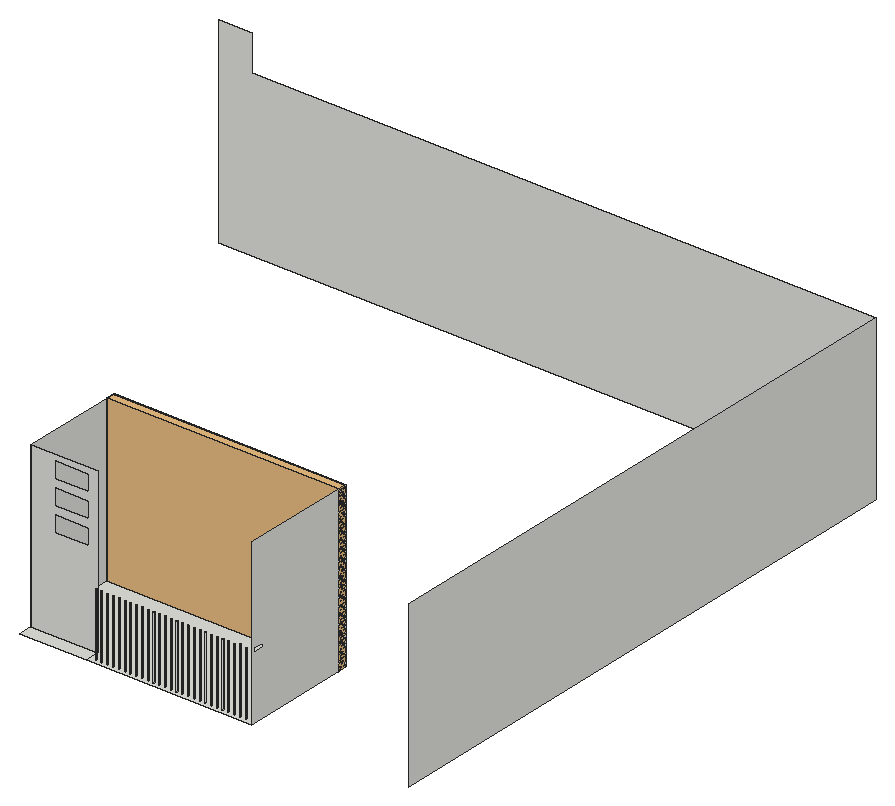
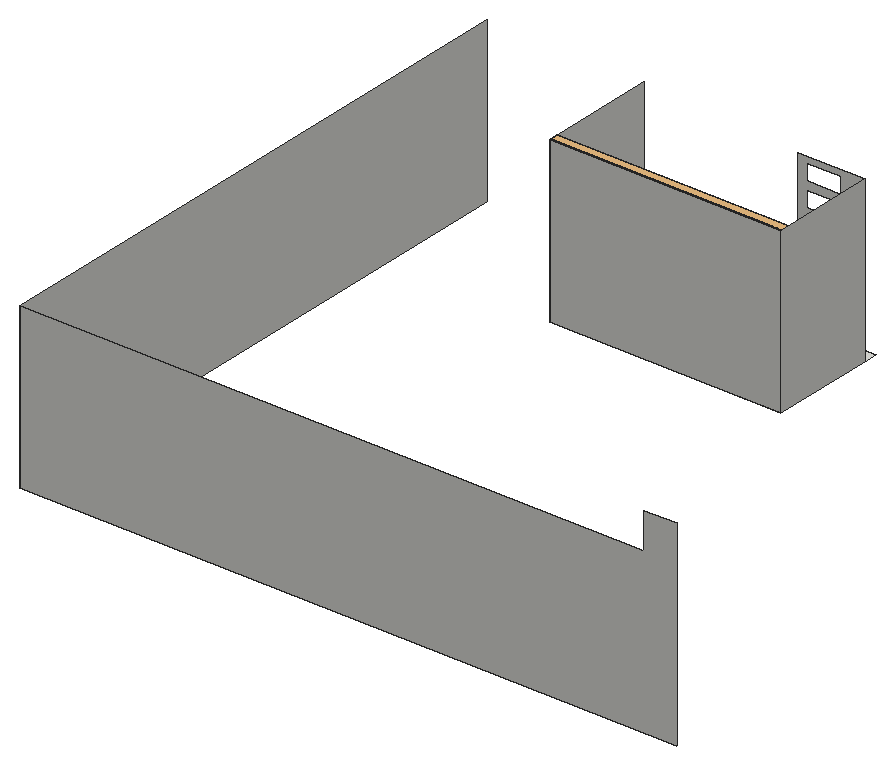
# SketchUp Ruby script. Lengths in inches.
U = 1.inch
M = Sketchup.active_model
def pt(a) = Geom::Point3d.new(a.map { |v| v * U })
def face(e, loops, mat)
  f = e.add_face(loops[0].map { |a| pt(a) })
  loops[1..].each { |l| e.add_face(l.map { |a| pt(a) }).erase! }
  f.material = f.back_material = mat if mat
  f
end
# faces: each face lists its corners as indices into pts; further lists are holes
def faces(e, pts, list, mat = nil) = list.each { |f| face(e, (f[0].is_a?(Array) ? f : [f]).map { |l| l.map { |i| pts[i] } }, mat) }
# xy, xz, yz: faces in a plane at the given z, y or x. An outline is a flat list of corners, or four numbers for a rectangle; further outlines are holes
def ring(l) = l.size == 4 ? [[l[0], l[1]], [l[2], l[1]], [l[2], l[3]], [l[0], l[3]]] : l.each_slice(2).to_a
def flat(e, list, mat, &to3) = list.each { |f| face(e, (f[0].is_a?(Array) ? f : [f]).map { |l| ring(l).map { |u, v| to3.(u, v) } }, mat) }
def xy(e, z, list, mat = nil) = flat(e, list, mat) { |x, y| [x, y, z] }
def xz(e, y, list, mat = nil) = flat(e, list, mat) { |x, z| [x, y, z] }
def yz(e, x, list, mat = nil) = flat(e, list, mat) { |y, z| [x, y, z] }
def lines(e, pts, list) = list.each { |a, b| e.add_line(pt(pts[a]), pt(pts[b])) }
# prism: a flat outline (further loops are holes) pulled along v
def prism(e, loops, v, mat = nil)
  f = face(e, loops, mat); d = Geom::Vector3d.new(v.map { |x| x * U })
  f.pushpull(f.normal.samedirection?(d) ? d.length : -d.length)
end
def box(e, o, s, mat = nil) = prism(e, [[o, [o[0] + s[0], o[1], o[2]], [o[0] + s[0], o[1] + s[1], o[2]], [o[0], o[1] + s[1], o[2]]]], [0, 0, s[2]], mat)
def at(x, y, z, deg = 0) = Geom::Transformation.translation(pt([x, y, z])) * Geom::Transformation.rotation(ORIGIN, Z_AXIS, deg.degrees)
def axes(o, x, y, z) = Geom::Transformation.new([*x, 0, *y, 0, *z, 0, *pt(o).to_a, 1])
def part(name) = M.definitions.add(name)
# library, detail: a bought-in or finely detailed component or shape, given as its bounding box
def library(name, o, s) = part(name).tap { |d| box(d.entities, o, s) }
def detail(e, o, s) = box(e.add_group.entities, o, s)
def put(e, d, t, mat = nil) = e.add_instance(d, t).tap { |i| i.material = mat if mat }
def group(e, t, mat = nil) = e.add_group.tap { |g| g.transformation = t; g.material = mat if mat }.entities
root = M.entities
c1 = library("Group\#10",[0,0,0],[238.3125,8.8125,168])
xy(root,819.75,[[290.4375,124.5,359.25,138.74],[[359.25,124.5,528.75,124.5,528.75,246,290.4375,246,290.4375,138.74,359.25,138.74],[370.76,127.81,370.55,127.83,370.35,127.91,370.1875,128.04,370.06,128.21,369.98,128.41,369.95,128.62,369.98,128.83,370.06,129.02,370.1875,129.19,370.35,129.32,370.55,129.4,370.76,129.43,370.97,129.4,371.17,129.32,371.34,129.19,371.46,129.02,371.55,128.83,371.57,128.62,371.55,128.41,371.46,128.21,371.34,128.04,371.17,127.91,370.97,127.83],[365.01,127.81,364.8,127.83,364.6,127.91,364.4375,128.04,364.31,128.21,364.23,128.41,364.2,128.62,364.23,128.83,364.31,129.02,364.4375,129.19,364.6,129.32,364.8,129.4,365.01,129.43,365.22,129.4,365.42,129.32,365.59,129.19,365.71,129.02,365.8,128.83,365.82,128.62,365.8,128.41,365.71,128.21,365.59,128.04,365.42,127.91,365.22,127.83],[376.7,127.81,376.49,127.83,376.29,127.91,376.125,128.04,375.99,128.21,375.91,128.41,375.89,128.62,375.91,128.83,375.99,129.02,376.125,129.19,376.29,129.32,376.49,129.4,376.7,129.43,376.91,129.4,377.1,129.32,377.27,129.19,377.4,129.02,377.48,128.83,377.51,128.62,377.48,128.41,377.4,128.21,377.27,128.04,377.1,127.91,376.91,127.83],[382.76,127.81,382.55,127.83,382.35,127.91,382.1875,128.04,382.06,128.21,381.98,128.41,381.95,128.62,381.98,128.83,382.06,129.02,382.1875,129.19,382.35,129.32,382.55,129.4,382.76,129.43,382.97,129.4,383.17,129.32,383.34,129.19,383.46,129.02,383.55,128.83,383.57,128.62,383.55,128.41,383.46,128.21,383.34,128.04,383.17,127.91,382.97,127.83],[388.82,127.81,388.61,127.83,388.42,127.91,388.25,128.04,388.12,128.21,388.04,128.41,388.01,128.62,388.04,128.83,388.12,129.02,388.25,129.19,388.42,129.32,388.61,129.4,388.82,129.43,389.03,129.4,389.23,129.32,389.4,129.19,389.53,129.02,389.61,128.83,389.64,128.62,389.61,128.41,389.53,128.21,389.4,128.04,389.23,127.91,389.03,127.83],[394.76,127.81,394.55,127.83,394.35,127.91,394.1875,128.04,394.06,128.21,393.98,128.41,393.95,128.62,393.98,128.83,394.06,129.02,394.1875,129.19,394.35,129.32,394.55,129.4,394.76,129.43,394.97,129.4,395.17,129.32,395.34,129.19,395.46,129.02,395.55,128.83,395.57,128.62,395.55,128.41,395.46,128.21,395.34,128.04,395.17,127.91,394.97,127.83],[400.57,127.81,400.36,127.83,400.17,127.91,400,128.04,399.87,128.21,399.79,128.41,399.76,128.62,399.79,128.83,399.87,129.02,400,129.19,400.17,129.32,400.36,129.4,400.57,129.43,400.78,129.4,400.98,129.32,401.15,129.19,401.28,129.02,401.36,128.83,401.39,128.62,401.36,128.41,401.28,128.21,401.15,128.04,400.98,127.91,400.78,127.83],[406.39,127.81,406.18,127.83,405.98,127.91,405.8125,128.04,405.68,128.21,405.6,128.41,405.57,128.62,405.6,128.83,405.68,129.02,405.8125,129.19,405.98,129.32,406.18,129.4,406.39,129.43,406.6,129.4,406.79,129.32,406.96,129.19,407.09,129.02,407.17,128.83,407.2,128.62,407.17,128.41,407.09,128.21,406.96,128.04,406.79,127.91,406.6,127.83],[412.32,127.81,412.11,127.83,411.92,127.91,411.75,128.04,411.62,128.21,411.54,128.41,411.51,128.62,411.54,128.83,411.62,129.02,411.75,129.19,411.92,129.32,412.11,129.4,412.32,129.43,412.53,129.4,412.73,129.32,412.9,129.19,413.03,129.02,413.11,128.83,413.14,128.62,413.11,128.41,413.03,128.21,412.9,128.04,412.73,127.91,412.53,127.83],[418.45,127.81,418.24,127.83,418.04,127.91,417.875,128.04,417.74,128.21,417.66,128.41,417.64,128.62,417.66,128.83,417.74,129.02,417.875,129.19,418.04,129.32,418.24,129.4,418.45,129.43,418.66,129.4,418.85,129.32,419.02,129.19,419.15,129.02,419.23,128.83,419.26,128.62,419.23,128.41,419.15,128.21,419.02,128.04,418.85,127.91,418.66,127.83],[424.39,127.81,424.18,127.83,423.98,127.91,423.8125,128.04,423.68,128.21,423.6,128.41,423.57,128.62,423.6,128.83,423.68,129.02,423.8125,129.19,423.98,129.32,424.18,129.4,424.39,129.43,424.6,129.4,424.79,129.32,424.96,129.19,425.09,129.02,425.17,128.83,425.2,128.62,425.17,128.41,425.09,128.21,424.96,128.04,424.79,127.91,424.6,127.83],[430.2,127.81,429.99,127.83,429.79,127.91,429.625,128.04,429.49,128.21,429.41,128.41,429.39,128.62,429.41,128.83,429.49,129.02,429.625,129.19,429.79,129.32,429.99,129.4,430.2,129.43,430.41,129.4,430.6,129.32,430.77,129.19,430.9,129.02,430.98,128.83,431.01,128.62,430.98,128.41,430.9,128.21,430.77,128.04,430.6,127.91,430.41,127.83],[436.01,127.81,435.8,127.83,435.6,127.91,435.4375,128.04,435.31,128.21,435.23,128.41,435.2,128.62,435.23,128.83,435.31,129.02,435.4375,129.19,435.6,129.32,435.8,129.4,436.01,129.43,436.22,129.4,436.42,129.32,436.59,129.19,436.71,129.02,436.8,128.83,436.82,128.62,436.8,128.41,436.71,128.21,436.59,128.04,436.42,127.91,436.22,127.83],[442.01,127.81,441.8,127.83,441.6,127.91,441.4375,128.04,441.31,128.21,441.23,128.41,441.2,128.62,441.23,128.83,441.31,129.02,441.4375,129.19,441.6,129.32,441.8,129.4,442.01,129.43,442.22,129.4,442.42,129.32,442.59,129.19,442.71,129.02,442.8,128.83,442.82,128.62,442.8,128.41,442.71,128.21,442.59,128.04,442.42,127.91,442.22,127.83],[448.07,127.81,447.86,127.83,447.67,127.91,447.5,128.04,447.37,128.21,447.29,128.41,447.26,128.62,447.29,128.83,447.37,129.02,447.5,129.19,447.67,129.32,447.86,129.4,448.07,129.43,448.28,129.4,448.48,129.32,448.65,129.19,448.78,129.02,448.86,128.83,448.89,128.62,448.86,128.41,448.78,128.21,448.65,128.04,448.48,127.91,448.28,127.83],[453.89,127.81,453.68,127.83,453.48,127.91,453.3125,128.04,453.18,128.21,453.1,128.41,453.07,128.62,453.1,128.83,453.18,129.02,453.3125,129.19,453.48,129.32,453.68,129.4,453.89,129.43,454.1,129.4,454.29,129.32,454.46,129.19,454.59,129.02,454.67,128.83,454.7,128.62,454.67,128.41,454.59,128.21,454.46,128.04,454.29,127.91,454.1,127.83],[459.95,127.81,459.74,127.83,459.54,127.91,459.375,128.04,459.24,128.21,459.16,128.41,459.14,128.62,459.16,128.83,459.24,129.02,459.375,129.19,459.54,129.32,459.74,129.4,459.95,129.43,460.16,129.4,460.35,129.32,460.52,129.19,460.65,129.02,460.73,128.83,460.76,128.62,460.73,128.41,460.65,128.21,460.52,128.04,460.35,127.91,460.16,127.83],[465.76,127.81,465.55,127.83,465.35,127.91,465.1875,128.04,465.06,128.21,464.98,128.41,464.95,128.62,464.98,128.83,465.06,129.02,465.1875,129.19,465.35,129.32,465.55,129.4,465.76,129.43,465.97,129.4,466.17,129.32,466.34,129.19,466.46,129.02,466.55,128.83,466.57,128.62,466.55,128.41,466.46,128.21,466.34,128.04,466.17,127.91,465.97,127.83],[471.95,127.81,471.74,127.83,471.54,127.91,471.375,128.04,471.24,128.21,471.16,128.41,471.14,128.62,471.16,128.83,471.24,129.02,471.375,129.19,471.54,129.32,471.74,129.4,471.95,129.43,472.16,129.4,472.35,129.32,472.52,129.19,472.65,129.02,472.73,128.83,472.76,128.62,472.73,128.41,472.65,128.21,472.52,128.04,472.35,127.91,472.16,127.83],[477.76,127.81,477.55,127.83,477.35,127.91,477.1875,128.04,477.06,128.21,476.98,128.41,476.95,128.62,476.98,128.83,477.06,129.02,477.1875,129.19,477.35,129.32,477.55,129.4,477.76,129.43,477.97,129.4,478.17,129.32,478.34,129.19,478.46,129.02,478.55,128.83,478.57,128.62,478.55,128.41,478.46,128.21,478.34,128.04,478.17,127.91,477.97,127.83],[483.76,127.81,483.55,127.83,483.35,127.91,483.1875,128.04,483.06,128.21,482.98,128.41,482.95,128.62,482.98,128.83,483.06,129.02,483.1875,129.19,483.35,129.32,483.55,129.4,483.76,129.43,483.97,129.4,484.17,129.32,484.34,129.19,484.46,129.02,484.55,128.83,484.57,128.62,484.55,128.41,484.46,128.21,484.34,128.04,484.17,127.91,483.97,127.83],[489.89,127.81,489.68,127.83,489.48,127.91,489.3125,128.04,489.18,128.21,489.1,128.41,489.07,128.62,489.1,128.83,489.18,129.02,489.3125,129.19,489.48,129.32,489.68,129.4,489.89,129.43,490.1,129.4,490.29,129.32,490.46,129.19,490.59,129.02,490.67,128.83,490.7,128.62,490.67,128.41,490.59,128.21,490.46,128.04,490.29,127.91,490.1,127.83],[495.39,127.81,495.18,127.83,494.98,127.91,494.8125,128.04,494.68,128.21,494.6,128.41,494.57,128.62,494.6,128.83,494.68,129.02,494.8125,129.19,494.98,129.32,495.18,129.4,495.39,129.43,495.6,129.4,495.79,129.32,495.96,129.19,496.09,129.02,496.17,128.83,496.2,128.62,496.17,128.41,496.09,128.21,495.96,128.04,495.79,127.91,495.6,127.83],[501.32,127.81,501.11,127.83,500.92,127.91,500.75,128.04,500.62,128.21,500.54,128.41,500.51,128.62,500.54,128.83,500.62,129.02,500.75,129.19,500.92,129.32,501.11,129.4,501.32,129.43,501.53,129.4,501.73,129.32,501.9,129.19,502.03,129.02,502.11,128.83,502.14,128.62,502.11,128.41,502.03,128.21,501.9,128.04,501.73,127.91,501.53,127.83],[507.39,127.81,507.18,127.83,506.98,127.91,506.8125,128.04,506.68,128.21,506.6,128.41,506.57,128.62,506.6,128.83,506.68,129.02,506.8125,129.19,506.98,129.32,507.18,129.4,507.39,129.43,507.6,129.4,507.79,129.32,507.96,129.19,508.09,129.02,508.17,128.83,508.2,128.62,508.17,128.41,508.09,128.21,507.96,128.04,507.79,127.91,507.6,127.83],[513.45,127.81,513.24,127.83,513.04,127.91,512.875,128.04,512.74,128.21,512.66,128.41,512.64,128.62,512.66,128.83,512.74,129.02,512.875,129.19,513.04,129.32,513.24,129.4,513.45,129.43,513.66,129.4,513.85,129.32,514.02,129.19,514.15,129.02,514.23,128.83,514.26,128.62,514.23,128.41,514.15,128.21,514.02,128.04,513.85,127.91,513.66,127.83],[519.32,127.81,519.11,127.83,518.92,127.91,518.75,128.04,518.62,128.21,518.54,128.41,518.51,128.62,518.54,128.83,518.62,129.02,518.75,129.19,518.92,129.32,519.11,129.4,519.32,129.43,519.53,129.4,519.73,129.32,519.9,129.19,520.03,129.02,520.11,128.83,520.14,128.62,520.11,128.41,520.03,128.21,519.9,128.04,519.73,127.91,519.53,127.83]]])
xz(root,138.74,[[[290.4375,819.75,359.25,987.75],[314.83,915.33,349.58,932.2],[314.83,940.2,349.58,957.08],[314.83,965.08,349.58,981.95]]])
xz(root,246,[[290.4375,819.75,528.75,987.75]])
xz(root,724.5,[[15.3125,819.75,15.3125,1024.6875,48.5,1024.6875,48.5,987.75,690.4375,987.75,690.4375,819.75]])
yz(root,290.4375,[[138.74,819.75,246,987.75]])
yz(root,528.75,[[[124.5,819.75,246,987.75],[127.31,884.89,138.74,889.08]]])
yz(root,690.4375,[[124.5,819.75,724.5,987.75]])
p = [[371.46,129.02,819.75],[371.34,129.19,819.75],[371.34,129.19,884.89],[371.46,129.02,884.89],[364.6,129.32,819.75],[364.4375,129.19,819.75],
  [364.4375,129.19,884.89],[364.6,129.32,884.89],[365.59,129.19,819.75],[365.42,129.32,819.75],[365.42,129.32,884.89],[365.59,129.19,884.89],
  [370.35,129.32,819.75],[370.1875,129.19,819.75],[370.1875,129.19,884.89],[370.35,129.32,884.89],[371.17,129.32,819.75],[371.17,129.32,884.89],
  [376.29,129.32,819.75],[376.125,129.19,819.75],[376.125,129.19,884.89],[376.29,129.32,884.89],[377.27,129.19,819.75],[377.1,129.32,819.75],
  [377.1,129.32,884.89],[377.27,129.19,884.89],[382.35,129.32,819.75],[382.1875,129.19,819.75],[382.1875,129.19,884.89],[382.35,129.32,884.89],
  [383.34,129.19,819.75],[383.17,129.32,819.75],[383.17,129.32,884.89],[383.34,129.19,884.89],[388.42,129.32,819.75],[388.25,129.19,819.75],
  [388.25,129.19,884.89],[388.42,129.32,884.89],[389.4,129.19,819.75],[389.23,129.32,819.75],[389.23,129.32,884.89],[389.4,129.19,884.89],
  [394.35,129.32,819.75],[394.1875,129.19,819.75],[394.1875,129.19,884.89],[394.35,129.32,884.89],[395.34,129.19,819.75],[395.17,129.32,819.75],
  [395.17,129.32,884.89],[395.34,129.19,884.89],[400.17,129.32,819.75],[400,129.19,819.75],[400,129.19,884.89],[400.17,129.32,884.89],
  [401.15,129.19,819.75],[400.98,129.32,819.75],[400.98,129.32,884.89],[401.15,129.19,884.89],[405.98,129.32,819.75],[405.8125,129.19,819.75],
  [405.8125,129.19,884.89],[405.98,129.32,884.89],[406.96,129.19,819.75],[406.79,129.32,819.75],[406.79,129.32,884.89],[406.96,129.19,884.89],
  [411.92,129.32,819.75],[411.75,129.19,819.75],[411.75,129.19,884.89],[411.92,129.32,884.89],[412.9,129.19,819.75],[412.73,129.32,819.75],
  [412.73,129.32,884.89],[412.9,129.19,884.89],[418.04,129.32,819.75],[417.875,129.19,819.75],[417.875,129.19,884.89],[418.04,129.32,884.89],
  [419.02,129.19,819.75],[418.85,129.32,819.75],[418.85,129.32,884.89],[419.02,129.19,884.89],[423.98,129.32,819.75],[423.8125,129.19,819.75],
  [423.8125,129.19,884.89],[423.98,129.32,884.89],[424.96,129.19,819.75],[424.79,129.32,819.75],[424.79,129.32,884.89],[424.96,129.19,884.89],
  [429.79,129.32,819.75],[429.625,129.19,819.75],[429.625,129.19,884.89],[429.79,129.32,884.89],[430.77,129.19,819.75],[430.6,129.32,819.75],
  [430.6,129.32,884.89],[430.77,129.19,884.89],[435.6,129.32,819.75],[435.4375,129.19,819.75],[435.4375,129.19,884.89],[435.6,129.32,884.89],
  [436.59,129.19,819.75],[436.42,129.32,819.75],[436.42,129.32,884.89],[436.59,129.19,884.89],[441.6,129.32,819.75],[441.4375,129.19,819.75],
  [441.4375,129.19,884.89],[441.6,129.32,884.89],[442.59,129.19,819.75],[442.42,129.32,819.75],[442.42,129.32,884.89],[442.59,129.19,884.89],
  [447.67,129.32,819.75],[447.5,129.19,819.75],[447.5,129.19,884.89],[447.67,129.32,884.89],[448.65,129.19,819.75],[448.48,129.32,819.75],
  [448.48,129.32,884.89],[448.65,129.19,884.89],[453.48,129.32,819.75],[453.3125,129.19,819.75],[453.3125,129.19,884.89],[453.48,129.32,884.89],
  [454.46,129.19,819.75],[454.29,129.32,819.75],[454.29,129.32,884.89],[454.46,129.19,884.89],[459.54,129.32,819.75],[459.375,129.19,819.75],
  [459.375,129.19,884.89],[459.54,129.32,884.89],[460.52,129.19,819.75],[460.35,129.32,819.75],[460.35,129.32,884.89],[460.52,129.19,884.89],
  [465.35,129.32,819.75],[465.1875,129.19,819.75],[465.1875,129.19,884.89],[465.35,129.32,884.89],[466.34,129.19,819.75],[466.17,129.32,819.75],
  [466.17,129.32,884.89],[466.34,129.19,884.89],[471.54,129.32,819.75],[471.375,129.19,819.75],[471.375,129.19,884.89],[471.54,129.32,884.89],
  [472.52,129.19,819.75],[472.35,129.32,819.75],[472.35,129.32,884.89],[472.52,129.19,884.89],[477.35,129.32,819.75],[477.1875,129.19,819.75],
  [477.1875,129.19,884.89],[477.35,129.32,884.89],[478.34,129.19,819.75],[478.17,129.32,819.75],[478.17,129.32,884.89],[478.34,129.19,884.89],
  [483.35,129.32,819.75],[483.1875,129.19,819.75],[483.1875,129.19,884.89],[483.35,129.32,884.89],[484.34,129.19,819.75],[484.17,129.32,819.75],
  [484.17,129.32,884.89],[484.34,129.19,884.89],[489.48,129.32,819.75],[489.3125,129.19,819.75],[489.3125,129.19,884.89],[489.48,129.32,884.89],
  [490.46,129.19,819.75],[490.29,129.32,819.75],[490.29,129.32,884.89],[490.46,129.19,884.89],[494.98,129.32,819.75],[494.8125,129.19,819.75],
  [494.8125,129.19,884.89],[494.98,129.32,884.89],[495.96,129.19,819.75],[495.79,129.32,819.75],[495.79,129.32,884.89],[495.96,129.19,884.89],
  [500.92,129.32,819.75],[500.75,129.19,819.75],[500.75,129.19,884.89],[500.92,129.32,884.89],[501.9,129.19,819.75],[501.73,129.32,819.75],
  [501.73,129.32,884.89],[501.9,129.19,884.89],[506.98,129.32,819.75],[506.8125,129.19,819.75],[506.8125,129.19,884.89],[506.98,129.32,884.89],
  [507.96,129.19,819.75],[507.79,129.32,819.75],[507.79,129.32,884.89],[507.96,129.19,884.89],[513.04,129.32,819.75],[512.875,129.19,819.75],
  [512.875,129.19,886.75],[513.04,129.32,886.75],[514.02,129.19,819.75],[513.85,129.32,819.75],[513.85,129.32,886.75],[514.02,129.19,886.75],
  [518.92,129.32,819.75],[518.75,129.19,819.75],[518.75,129.19,884.89],[518.92,129.32,884.89],[519.9,129.19,819.75],[519.73,129.32,819.75],
  [519.73,129.32,884.89],[519.9,129.19,884.89],[364.8,129.4,819.75],[364.8,129.4,884.89],[365.22,129.4,819.75],[365.22,129.4,884.89],
  [370.55,129.4,819.75],[370.55,129.4,884.89],[370.97,129.4,819.75],[370.97,129.4,884.89],[376.49,129.4,819.75],[376.49,129.4,884.89],
  [376.91,129.4,819.75],[376.91,129.4,884.89],[382.55,129.4,819.75],[382.55,129.4,884.89],[382.97,129.4,819.75],[382.97,129.4,884.89],
  [388.61,129.4,819.75],[388.61,129.4,884.89],[389.03,129.4,819.75],[389.03,129.4,884.89],[394.55,129.4,819.75],[394.55,129.4,884.89],
  [394.97,129.4,819.75],[394.97,129.4,884.89],[400.36,129.4,819.75],[400.36,129.4,884.89],[400.78,129.4,819.75],[400.78,129.4,884.89],
  [406.18,129.4,819.75],[406.18,129.4,884.89],[406.6,129.4,819.75],[406.6,129.4,884.89],[412.11,129.4,819.75],[412.11,129.4,884.89],
  [412.53,129.4,819.75],[412.53,129.4,884.89],[418.24,129.4,819.75],[418.24,129.4,884.89],[418.66,129.4,819.75],[418.66,129.4,884.89],
  [424.18,129.4,819.75],[424.18,129.4,884.89],[424.6,129.4,819.75],[424.6,129.4,884.89],[429.99,129.4,819.75],[429.99,129.4,884.89],
  [430.41,129.4,819.75],[430.41,129.4,884.89],[435.8,129.4,819.75],[435.8,129.4,884.89],[436.22,129.4,819.75],[436.22,129.4,884.89],
  [441.8,129.4,819.75],[441.8,129.4,884.89],[442.22,129.4,819.75],[442.22,129.4,884.89],[447.86,129.4,819.75],[447.86,129.4,884.89],
  [448.28,129.4,819.75],[448.28,129.4,884.89],[453.68,129.4,819.75],[453.68,129.4,884.89],[454.1,129.4,819.75],[454.1,129.4,884.89],
  [459.74,129.4,819.75],[459.74,129.4,884.89],[460.16,129.4,819.75],[460.16,129.4,884.89],[465.55,129.4,819.75],[465.55,129.4,884.89],
  [465.97,129.4,819.75],[465.97,129.4,884.89],[471.74,129.4,819.75],[471.74,129.4,884.89],[472.16,129.4,819.75],[472.16,129.4,884.89],
  [477.55,129.4,819.75],[477.55,129.4,884.89],[477.97,129.4,819.75],[477.97,129.4,884.89],[483.55,129.4,819.75],[483.55,129.4,884.89],
  [483.97,129.4,819.75],[483.97,129.4,884.89],[489.68,129.4,819.75],[489.68,129.4,884.89],[490.1,129.4,819.75],[490.1,129.4,884.89],
  [495.18,129.4,819.75],[495.18,129.4,884.89],[495.6,129.4,819.75],[495.6,129.4,884.89],[501.11,129.4,819.75],[501.11,129.4,884.89],
  [501.53,129.4,819.75],[501.53,129.4,884.89],[507.18,129.4,819.75],[507.18,129.4,884.89],[507.6,129.4,819.75],[507.6,129.4,884.89],
  [513.24,129.4,819.75],[513.24,129.4,886.75],[513.66,129.4,819.75],[513.66,129.4,886.75],[519.11,129.4,819.75],[519.11,129.4,884.89],
  [519.53,129.4,819.75],[519.53,129.4,884.89],[365.01,129.43,819.75],[365.01,129.43,884.89],[370.76,129.43,819.75],[370.76,129.43,884.89],
  [376.7,129.43,819.75],[376.7,129.43,884.89],[382.76,129.43,819.75],[382.76,129.43,884.89],[388.82,129.43,819.75],[388.82,129.43,884.89],
  [394.76,129.43,819.75],[394.76,129.43,884.89],[400.57,129.43,819.75],[400.57,129.43,884.89],[406.39,129.43,819.75],[406.39,129.43,884.89],
  [412.32,129.43,819.75],[412.32,129.43,884.89],[418.45,129.43,819.75],[418.45,129.43,884.89],[424.39,129.43,819.75],[424.39,129.43,884.89],
  [430.2,129.43,819.75],[430.2,129.43,884.89],[436.01,129.43,819.75],[436.01,129.43,884.89],[442.01,129.43,819.75],[442.01,129.43,884.89],
  [448.07,129.43,819.75],[448.07,129.43,884.89],[453.89,129.43,819.75],[453.89,129.43,884.89],[459.95,129.43,819.75],[459.95,129.43,884.89],
  [465.76,129.43,819.75],[465.76,129.43,884.89],[471.95,129.43,819.75],[471.95,129.43,884.89],[477.76,129.43,819.75],[477.76,129.43,884.89],
  [483.76,129.43,819.75],[483.76,129.43,884.89],[489.89,129.43,819.75],[489.89,129.43,884.89],[495.39,129.43,819.75],[495.39,129.43,884.89],
  [501.32,129.43,819.75],[501.32,129.43,884.89],[507.39,129.43,819.75],[507.39,129.43,884.89],[513.45,129.43,819.75],[513.45,129.43,886.75],
  [519.32,129.43,819.75],[519.32,129.43,884.89]]
faces(root,p,[[0,1,2,3],[4,5,6,7],[8,9,10,11],[12,13,14,15],[1,16,17,2],[18,19,20,21],[22,23,24,25],[26,27,28,29],
  [30,31,32,33],[34,35,36,37],[38,39,40,41],[42,43,44,45],[46,47,48,49],[50,51,52,53],[54,55,56,57],[58,59,60,61],
  [62,63,64,65],[66,67,68,69],[70,71,72,73],[74,75,76,77],[78,79,80,81],[82,83,84,85],[86,87,88,89],[90,91,92,93],
  [94,95,96,97],[98,99,100,101],[102,103,104,105],[106,107,108,109],[110,111,112,113],[114,115,116,117],[118,119,120,121],[122,123,124,125],
  [126,127,128,129],[130,131,132,133],[134,135,136,137],[138,139,140,141],[142,143,144,145],[146,147,148,149],[150,151,152,153],[154,155,156,157],
  [158,159,160,161],[162,163,164,165],[166,167,168,169],[170,171,172,173],[174,175,176,177],[178,179,180,181],[182,183,184,185],[186,187,188,189],
  [190,191,192,193],[194,195,196,197],[198,199,200,201],[202,203,204,205],[206,207,208,209],[210,211,212,213],[214,215,216,217],[218,4,7,219],
  [9,220,221,10],[222,12,15,223],[16,224,225,17],[226,18,21,227],[23,228,229,24],[230,26,29,231],[31,232,233,32],[234,34,37,235],
  [39,236,237,40],[238,42,45,239],[47,240,241,48],[242,50,53,243],[55,244,245,56],[246,58,61,247],[63,248,249,64],[250,66,69,251],
  [71,252,253,72],[254,74,77,255],[79,256,257,80],[258,82,85,259],[87,260,261,88],[262,90,93,263],[95,264,265,96],[266,98,101,267],
  [103,268,269,104],[270,106,109,271],[111,272,273,112],[274,114,117,275],[119,276,277,120],[278,122,125,279],[127,280,281,128],[282,130,133,283],
  [135,284,285,136],[286,138,141,287],[143,288,289,144],[290,146,149,291],[151,292,293,152],[294,154,157,295],[159,296,297,160],[298,162,165,299],
  [167,300,301,168],[302,170,173,303],[175,304,305,176],[306,178,181,307],[183,308,309,184],[310,186,189,311],[191,312,313,192],[314,194,197,315],
  [199,316,317,200],[318,202,205,319],[207,320,321,208],[322,210,213,323],[215,324,325,216],[326,218,219,327],[220,326,327,221],[328,222,223,329],
  [224,328,329,225],[330,226,227,331],[228,330,331,229],[332,230,231,333],[232,332,333,233],[334,234,235,335],[236,334,335,237],[336,238,239,337],
  [240,336,337,241],[338,242,243,339],[244,338,339,245],[340,246,247,341],[248,340,341,249],[342,250,251,343],[252,342,343,253],[344,254,255,345],
  [256,344,345,257],[346,258,259,347],[260,346,347,261],[348,262,263,349],[264,348,349,265],[350,266,267,351],[268,350,351,269],[352,270,271,353],
  [272,352,353,273],[354,274,275,355],[276,354,355,277],[356,278,279,357],[280,356,357,281],[358,282,283,359],[284,358,359,285],[360,286,287,361],
  [288,360,361,289],[362,290,291,363],[292,362,363,293],[364,294,295,365],[296,364,365,297],[366,298,299,367],[300,366,367,301],[368,302,303,369],
  [304,368,369,305],[370,306,307,371],[308,370,371,309],[372,310,311,373],[312,372,373,313],[374,314,315,375],[316,374,375,317],[376,318,319,377],
  [320,376,377,321],[378,322,323,379],[324,378,379,325]])
put(root,c1,at(290.4375,236.03,819.75))
